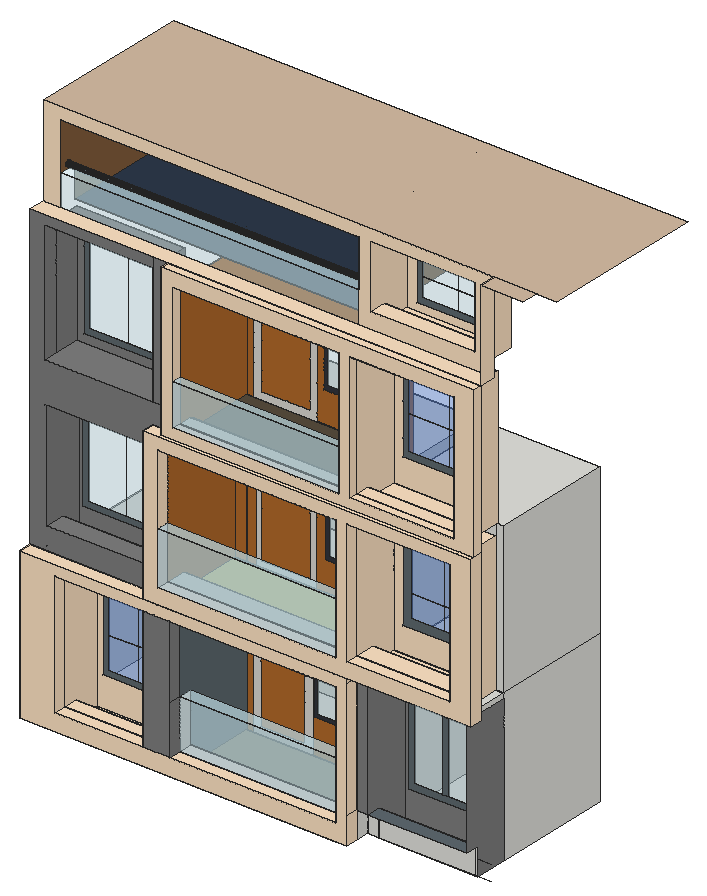
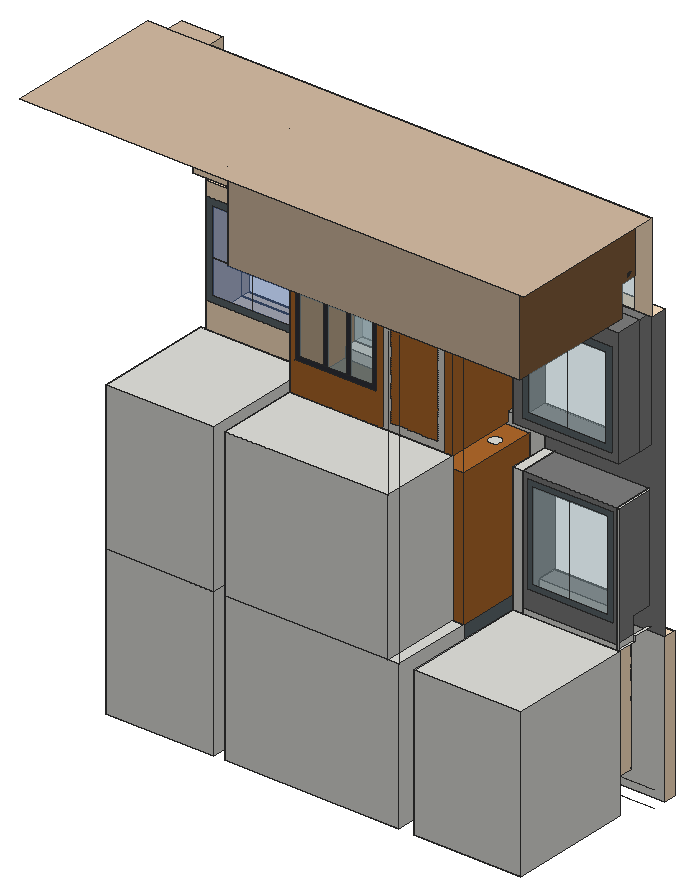
# SketchUp Ruby script. Lengths in inches.
U = 1.inch
M = Sketchup.active_model
def pt(a) = Geom::Point3d.new(a.map { |v| v * U })
def face(e, loops, mat)
  f = e.add_face(loops[0].map { |a| pt(a) })
  loops[1..].each { |l| e.add_face(l.map { |a| pt(a) }).erase! }
  f.material = f.back_material = mat if mat
  f
end
# faces: each face lists its corners as indices into pts; further lists are holes
def faces(e, pts, list, mat = nil) = list.each { |f| face(e, (f[0].is_a?(Array) ? f : [f]).map { |l| l.map { |i| pts[i] } }, mat) }
# xy, xz, yz: faces in a plane at the given z, y or x. An outline is a flat list of corners, or four numbers for a rectangle; further outlines are holes
def ring(l) = l.size == 4 ? [[l[0], l[1]], [l[2], l[1]], [l[2], l[3]], [l[0], l[3]]] : l.each_slice(2).to_a
def flat(e, list, mat, &to3) = list.each { |f| face(e, (f[0].is_a?(Array) ? f : [f]).map { |l| ring(l).map { |u, v| to3.(u, v) } }, mat) }
def xy(e, z, list, mat = nil) = flat(e, list, mat) { |x, y| [x, y, z] }
def xz(e, y, list, mat = nil) = flat(e, list, mat) { |x, z| [x, y, z] }
def yz(e, x, list, mat = nil) = flat(e, list, mat) { |y, z| [x, y, z] }
def lines(e, pts, list) = list.each { |a, b| e.add_line(pt(pts[a]), pt(pts[b])) }
# prism: a flat outline (further loops are holes) pulled along v
def prism(e, loops, v, mat = nil)
  f = face(e, loops, mat); d = Geom::Vector3d.new(v.map { |x| x * U })
  f.pushpull(f.normal.samedirection?(d) ? d.length : -d.length)
end
def box(e, o, s, mat = nil) = prism(e, [[o, [o[0] + s[0], o[1], o[2]], [o[0] + s[0], o[1] + s[1], o[2]], [o[0], o[1] + s[1], o[2]]]], [0, 0, s[2]], mat)
def at(x, y, z, deg = 0) = Geom::Transformation.translation(pt([x, y, z])) * Geom::Transformation.rotation(ORIGIN, Z_AXIS, deg.degrees)
def axes(o, x, y, z) = Geom::Transformation.new([*x, 0, *y, 0, *z, 0, *pt(o).to_a, 1])
def part(name) = M.definitions.add(name)
# library, detail: a bought-in or finely detailed component or shape, given as its bounding box
def library(name, o, s) = part(name).tap { |d| box(d.entities, o, s) }
def detail(e, o, s) = box(e.add_group.entities, o, s)
def put(e, d, t, mat = nil) = e.add_instance(d, t).tap { |i| i.material = mat if mat }
def group(e, t, mat = nil) = e.add_group.tap { |g| g.transformation = t; g.material = mat if mat }.entities
root = M.entities
M.materials.add("[0012_Bisque]").color = [255, 228, 196]
M.materials.add("[Blinds Wood Bamboo]").color = [131, 94, 60]
M.materials.add("[Carpet Diamond Olive]").color = [87, 77, 61]
M.materials.add("[Carpet Diamond Yellow]").color = [226, 217, 124]
M.materials.add("[Carpet Pattern Squares Multi]").color = [138, 129, 101]
M.materials.add("[Formica Laminate Dark]").color = [50, 53, 60]
M.materials.add("[Formica Laminate Light]").color = [213, 189, 164]
M.materials.add("[Formica Speckled Grey]").color = [94, 105, 111]
M.materials.add("[Leather Blue]").color = [45, 57, 74]
M.materials.add("[Slate Light Tile]").color = [127, 127, 127]
M.materials.add("[Terrazzo Tile Light]").color = [219, 217, 210]
M.materials.add("[Translucent Glass Blue]").color = [100, 149, 237]
M.materials["[Translucent Glass Blue]"].alpha = 0.5
M.materials.add("[Translucent Glass Safety]").color = [204, 235, 244]
M.materials["[Translucent Glass Safety]"].alpha = 0.5
M.materials.add("[Wood Bamboo]").color = [177, 105, 43]
xy(root,261,[[88.29,172.05,340.5,181.99],[340.5,172.05,349.51,181.99],[349.51,192.98,358.38,218.5],[99.28,214.18,186.23,314.81],[349.51,218.5,437.4,314.81],
  [198.44,249.06,340.5,314.81]])
xy(root,261,[[116.04,192.98,186.23,214.18]],"[0012_Bisque]")
xy(root,261,[[207.7,192.98,340.5,249.06]],"[Carpet Pattern Squares Multi]")
xy(root,261,[[358.38,192.98,437.4,218.5]],"[Formica Speckled Grey]")
xy(root,274.625,[[186.23,172.05,207.7,192.98],[207.7,181.99,340.5,192.98]])
xy(root,274.625,[[116.04,172.05,186.23,181.99],[207.7,172.05,340.5,181.99],[116.04,181.99,186.23,192.98]],"[0012_Bisque]")
xy(root,282.375,[[349.51,181.99,358.38,192.98]])
xy(root,282.375,[[358.38,181.99,437.4,192.98]],"[Formica Speckled Grey]")
xy(root,313.9375,[[207.7,181.99,340.5,192.98]],"[Translucent Glass Safety]")
xy(root,372.1875,[[222.36,205.33,221.21,205.48,220.14,205.93,219.22,206.63,218.51,207.55,218.07,208.62,217.92,209.77,218.07,210.92,218.51,211.99,219.22,212.91,220.14,213.61,221.21,214.05,222.36,214.21,223.51,214.05,224.58,213.61,225.5,212.91,226.2,211.99,226.64,210.92,226.8,209.77,226.64,208.62,226.2,207.55,225.5,206.63,224.58,205.93,223.51,205.48],[268.8,205.33,267.65,205.48,266.58,205.93,265.66,206.63,264.95,207.55,264.51,208.62,264.36,209.77,264.51,210.92,264.95,211.99,265.66,212.91,266.58,213.61,267.65,214.05,268.8,214.21,269.94,214.05,271.01,213.61,271.93,212.91,272.64,211.99,273.08,210.92,273.23,209.77,273.08,208.62,272.64,207.55,271.93,206.63,271.01,205.93,269.94,205.48],[320.23,205.33,319.08,205.48,318.01,205.93,317.1,206.63,316.39,207.55,315.95,208.62,315.8,209.77,315.95,210.92,316.39,211.99,317.1,212.91,318.01,213.61,319.08,214.05,320.23,214.21,321.38,214.05,322.45,213.61,323.37,212.91,324.08,211.99,324.52,210.92,324.67,209.77,324.52,208.62,324.08,207.55,323.37,206.63,322.45,205.93,321.38,205.48]])
xy(root,372.1875,[[116.04,172.05,186.23,181.99],[207.7,172.05,340.5,181.99],[116.04,181.99,186.23,214.18]],"[0012_Bisque]")
xy(root,372.1875,[[[207.7,181.99,340.5,249.06],[320.23,205.33,321.38,205.48,322.45,205.93,323.37,206.63,324.08,207.55,324.52,208.62,324.67,209.77,324.52,210.92,324.08,211.99,323.37,212.91,322.45,213.61,321.38,214.05,320.23,214.21,319.08,214.05,318.01,213.61,317.1,212.91,316.39,211.99,315.95,210.92,315.8,209.77,315.95,208.62,316.39,207.55,317.1,206.63,318.01,205.93,319.08,205.48],[222.36,205.33,223.51,205.48,224.58,205.93,225.5,206.63,226.2,207.55,226.64,208.62,226.8,209.77,226.64,210.92,226.2,211.99,225.5,212.91,224.58,213.61,223.51,214.05,222.36,214.21,221.21,214.05,220.14,213.61,219.22,212.91,218.51,211.99,218.07,210.92,217.92,209.77,218.07,208.62,218.51,207.55,219.22,206.63,220.14,205.93,221.21,205.48],[268.8,205.33,269.94,205.48,271.01,205.93,271.93,206.63,272.64,207.55,273.08,208.62,273.23,209.77,273.08,210.92,272.64,211.99,271.93,212.91,271.01,213.61,269.94,214.05,268.8,214.21,267.65,214.05,266.58,213.61,265.66,212.91,264.95,211.99,264.51,210.92,264.36,209.77,264.51,208.62,264.95,207.55,265.66,206.63,266.58,205.93,267.65,205.48]]],"[Wood Bamboo]")
xy(root,376.82,[[349.51,181.99,358.38,218.5]])
xy(root,376.82,[[358.38,181.99,437.4,218.5]],"[Slate Light Tile]")
xy(root,381,[[186.23,171.93,198.44,172.05],[198.44,171.93,340.5,172.05],[186.23,172.05,198.44,181.99],[198.44,172.05,340.5,181.99],[340.5,172.05,349.51,181.99],
  [198.44,181.99,431.53,198.09],[431.53,181.99,437.4,198.09],[99.8,198.09,101.61,214.18],[178.3,198.09,186.23,214.18],[431.53,198.09,437.4,218.5],
  [99.28,214.18,186.23,314.81],[349.51,218.5,437.4,314.81],[198.44,249.06,207.7,314.81],[207.7,249.06,340.5,314.81]])
xy(root,381,[[340.5,171.93,340.5,172.05,349.51,172.05,349.51,181.99,431.53,181.99,431.53,171.93],[431.53,171.93,437.4,181.99],[437.4,171.93,448.4,181.99],[88.29,172.05,186.23,181.99],[349.51,198.09,431.53,218.5]],"[0012_Bisque]")
xy(root,381,[[198.44,198.09,340.5,249.06]],"[Carpet Diamond Yellow]")
xy(root,384.875,[[99.8,181.99,101.61,198.09],[178.3,181.99,186.23,198.09]])
xy(root,384.875,[[101.61,198.09,178.3,214.18]],"[Slate Light Tile]")
xy(root,392.9375,[[198.44,171.93,340.5,181.99],[198.44,181.99,340.5,198.09]])
xy(root,392.9375,[[349.51,171.93,431.53,181.99],[349.51,181.99,431.53,198.09]],"[0012_Bisque]")
xy(root,399.125,[[101.61,181.99,178.3,198.09]],"[Slate Light Tile]")
xy(root,435,[[198.44,171.93,340.5,181.99]],"[Translucent Glass Safety]")
xy(root,485.17,[[99.8,181.99,101.61,214.18],[178.3,181.99,186.23,214.18]])
xy(root,485.17,[[101.61,181.99,178.3,214.18]],"[Slate Light Tile]")
xy(root,491.69,[[209.48,199,208.35,199.15,207.29,199.58,206.38,200.28,205.6875,201.1875,205.25,202.24,205.1,203.375,205.25,204.51,205.6875,205.5625,206.38,206.47,207.29,207.16,208.35,207.6,209.48,207.75,210.61,207.6,211.67,207.16,212.57,206.47,213.27,205.5625,213.7,204.51,213.85,203.375,213.7,202.24,213.27,201.1875,212.57,200.28,211.67,199.58,210.61,199.15],[260.29,199,259.16,199.15,258.1,199.58,257.2,200.28,256.5,201.1875,256.06,202.24,255.92,203.375,256.06,204.51,256.5,205.5625,257.2,206.47,258.1,207.16,259.16,207.6,260.29,207.75,261.42,207.6,262.48,207.16,263.38,206.47,264.08,205.5625,264.52,204.51,264.67,203.375,264.52,202.24,264.08,201.1875,263.38,200.28,262.48,199.58,261.42,199.15],[317.04,199,315.91,199.15,314.85,199.58,313.95,200.28,313.25,201.1875,312.81,202.24,312.67,203.375,312.81,204.51,313.25,205.5625,313.95,206.47,314.85,207.16,315.91,207.6,317.04,207.75,318.17,207.6,319.23,207.16,320.13,206.47,320.83,205.5625,321.27,204.51,321.42,203.375,321.27,202.24,320.83,201.1875,320.13,200.28,319.23,199.58,318.17,199.15]])
xy(root,491.69,[[198.44,171.93,340.5,181.99],[349.51,171.93,431.53,181.99],[349.51,181.99,431.53,218.5]],"[0012_Bisque]")
xy(root,491.69,[[[198.44,181.99,340.5,249.06],[209.48,199,210.61,199.15,211.67,199.58,212.57,200.28,213.27,201.1875,213.7,202.24,213.85,203.375,213.7,204.51,213.27,205.5625,212.57,206.47,211.67,207.16,210.61,207.6,209.48,207.75,208.35,207.6,207.29,207.16,206.38,206.47,205.6875,205.5625,205.25,204.51,205.1,203.375,205.25,202.24,205.6875,201.1875,206.38,200.28,207.29,199.58,208.35,199.15],[317.04,199,318.17,199.15,319.23,199.58,320.13,200.28,320.83,201.1875,321.27,202.24,321.42,203.375,321.27,204.51,320.83,205.5625,320.13,206.47,319.23,207.16,318.17,207.6,317.04,207.75,315.91,207.6,314.85,207.16,313.95,206.47,313.25,205.5625,312.81,204.51,312.67,203.375,312.81,202.24,313.25,201.1875,313.95,200.28,314.85,199.58,315.91,199.15],[260.29,199,261.42,199.15,262.48,199.58,263.38,200.28,264.08,201.1875,264.52,202.24,264.67,203.375,264.52,204.51,264.08,205.5625,263.38,206.47,262.48,207.16,261.42,207.6,260.29,207.75,259.16,207.6,258.1,207.16,257.2,206.47,256.5,205.5625,256.06,204.51,255.92,203.375,256.06,202.24,256.5,201.1875,257.2,200.28,258.1,199.58,259.16,199.15]]],"[Wood Bamboo]")
xy(root,501,[[198.44,175.18,437.4,181.99],[437.4,175.18,448.4,181.99],[349.51,218.5,437.4,314.81],[207.7,249.06,340.5,314.81]])
xy(root,501,[[186.23,171.93,198.44,181.99],[198.44,171.93,437.4,175.18],[437.4,171.93,448.4,175.18],[349.51,193.01,431.53,218.5],[431.53,193.01,432.73,218.5]],"[0012_Bisque]")
xy(root,501,[[207.7,193.01,340.5,249.06]],"[Carpet Diamond Olive]")
xy(root,509,[[207.7,175.18,340.5,181.99],[207.7,181.99,340.5,193.01]])
xy(root,509,[[349.51,175.18,432.73,181.99],[349.51,181.99,432.73,193.01]],"[0012_Bisque]")
xy(root,517.375,[[99.8,181.99,186.23,214.18]],"[Slate Light Tile]")
xy(root,542.5,[[207.7,175.18,340.5,181.99]],"[Translucent Glass Safety]")
xy(root,609.93,[[226.8,191.29,225.88,191.42,225.02,191.77,224.28,192.34,223.72,193.08,223.36,193.93,223.24,194.86,223.36,195.78,223.72,196.64,224.28,197.375,225.02,197.94,225.88,198.3,226.8,198.42,227.73,198.3,228.58,197.94,229.32,197.375,229.89,196.64,230.24,195.78,230.37,194.86,230.24,193.93,229.89,193.08,229.32,192.34,228.58,191.77,227.73,191.42],[275.55,191.29,274.63,191.42,273.77,191.77,273.03,192.34,272.47,193.08,272.11,193.93,271.99,194.86,272.11,195.78,272.47,196.64,273.03,197.375,273.77,197.94,274.63,198.3,275.55,198.42,276.48,198.3,277.33,197.94,278.07,197.375,278.64,196.64,278.99,195.78,279.12,194.86,278.99,193.93,278.64,193.08,278.07,192.34,277.33,191.77,276.48,191.42],[316.55,191.29,315.63,191.42,314.77,191.77,314.03,192.34,313.47,193.08,313.11,193.93,312.99,194.86,313.11,195.78,313.47,196.64,314.03,197.375,314.77,197.94,315.63,198.3,316.55,198.42,317.48,198.3,318.33,197.94,319.07,197.375,319.64,196.64,319.99,195.78,320.12,194.86,319.99,193.93,319.64,193.08,319.07,192.34,318.33,191.77,317.48,191.42]])
xy(root,609.93,[[207.7,175.18,340.5,181.99]],"[0012_Bisque]")
xy(root,609.93,[[[207.7,181.99,340.5,249.06],[316.55,191.29,317.48,191.42,318.33,191.77,319.07,192.34,319.64,193.08,319.99,193.93,320.12,194.86,319.99,195.78,319.64,196.64,319.07,197.375,318.33,197.94,317.48,198.3,316.55,198.42,315.63,198.3,314.77,197.94,314.03,197.375,313.47,196.64,313.11,195.78,312.99,194.86,313.11,193.93,313.47,193.08,314.03,192.34,314.77,191.77,315.63,191.42],[226.8,191.29,227.73,191.42,228.58,191.77,229.32,192.34,229.89,193.08,230.24,193.93,230.37,194.86,230.24,195.78,229.89,196.64,229.32,197.375,228.58,197.94,227.73,198.3,226.8,198.42,225.88,198.3,225.02,197.94,224.28,197.375,223.72,196.64,223.36,195.78,223.24,194.86,223.36,193.93,223.72,193.08,224.28,192.34,225.02,191.77,225.88,191.42],[275.55,191.29,276.48,191.42,277.33,191.77,278.07,192.34,278.64,193.08,278.99,193.93,279.12,194.86,278.99,195.78,278.64,196.64,278.07,197.375,277.33,197.94,276.48,198.3,275.55,198.42,274.63,198.3,273.77,197.94,273.03,197.375,272.47,196.64,272.11,195.78,271.99,194.86,272.11,193.93,272.47,193.08,273.03,192.34,273.77,191.77,274.63,191.42]]],"[Wood Bamboo]")
xy(root,610.28,[[349.51,175.18,432.73,181.99],[349.51,181.99,432.73,218.5]],"[0012_Bisque]")
xy(root,613.53,[[99.8,181.99,186.23,193.01],[99.8,193.01,186.23,214.18]],"[Slate Light Tile]")
xy(root,621,[[198.44,175.18,448.4,181.99],[88.29,181.99,448.4,195.54],[349.51,209.22,432.73,231.625]],"[0012_Bisque]")
xy(root,621,[[101.84,209.22,340.5,312.25]],"[Leather Blue]")
xy(root,633.5,[[349.51,195.54,432.73,209.22]],"[0012_Bisque]")
xy(root,645.8125,[[101.84,195.54,340.5,209.22]],"[Translucent Glass Safety]")
xy(root,683.72,[[126.93,241.64,125.08,241.88,123.37,242.59,121.89,243.72,120.76,245.2,120.05,246.92,119.8,248.76,120.05,250.61,120.76,252.33,121.89,253.8,123.37,254.93,125.08,255.64,126.93,255.89,128.77,255.64,130.49,254.93,131.97,253.8,133.1,252.33,133.8125,250.61,134.05,248.76,133.8125,246.92,133.1,245.2,131.97,243.72,130.49,242.59,128.77,241.88],[220.12,241.64,218.27,241.88,216.55,242.59,215.08,243.72,213.95,245.2,213.23,246.92,212.99,248.76,213.23,250.61,213.95,252.33,215.08,253.8,216.55,254.93,218.27,255.64,220.12,255.89,221.96,255.64,223.68,254.93,225.15,253.8,226.29,252.33,227,250.61,227.24,248.76,227,246.92,226.29,245.2,225.15,243.72,223.68,242.59,221.96,241.88],[310.74,241.64,308.9,241.88,307.18,242.59,305.7,243.72,304.57,245.2,303.86,246.92,303.62,248.76,303.86,250.61,304.57,252.33,305.7,253.8,307.18,254.93,308.9,255.64,310.74,255.89,312.59,255.64,314.3,254.93,315.78,253.8,316.91,252.33,317.625,250.61,317.87,248.76,317.625,246.92,316.91,245.2,315.78,243.72,314.3,242.59,312.59,241.88]])
xy(root,683.72,[[349.51,195.54,432.73,231.625]],"[0012_Bisque]")
xy(root,683.72,[[[101.84,195.54,340.5,312.25],[126.93,241.64,128.77,241.88,130.49,242.59,131.97,243.72,133.1,245.2,133.8125,246.92,134.05,248.76,133.8125,250.61,133.1,252.33,131.97,253.8,130.49,254.93,128.77,255.64,126.93,255.89,125.08,255.64,123.37,254.93,121.89,253.8,120.76,252.33,120.05,250.61,119.8,248.76,120.05,246.92,120.76,245.2,121.89,243.72,123.37,242.59,125.08,241.88],[310.74,241.64,312.59,241.88,314.3,242.59,315.78,243.72,316.91,245.2,317.625,246.92,317.87,248.76,317.625,250.61,316.91,252.33,315.78,253.8,314.3,254.93,312.59,255.64,310.74,255.89,308.9,255.64,307.18,254.93,305.7,253.8,304.57,252.33,303.86,250.61,303.62,248.76,303.86,246.92,304.57,245.2,305.7,243.72,307.18,242.59,308.9,241.88],[220.12,241.64,221.96,241.88,223.68,242.59,225.15,243.72,226.29,245.2,227,246.92,227.24,248.76,227,250.61,226.29,252.33,225.15,253.8,223.68,254.93,221.96,255.64,220.12,255.89,218.27,255.64,216.55,254.93,215.08,253.8,213.95,252.33,213.23,250.61,212.99,248.76,213.23,246.92,213.95,245.2,215.08,243.72,216.55,242.59,218.27,241.88]]],"[Blinds Wood Bamboo]")
xy(root,693,[[448.4,181.99,482.08,195.54],[88.29,195.54,498.52,325.8]],"[Formica Laminate Light]")
xz(root,171.93,[[[186.23,381,448.4,501],[198.44,392.9375,340.5,491.69],[349.51,392.9375,431.53,491.69]]],"[0012_Bisque]")
xz(root,171.93,[[198.44,392.9375,340.5,435]],"[Translucent Glass Safety]")
xz(root,172.05,[[[88.29,261,349.51,381],[116.04,274.625,340.5,372.1875]]],"[0012_Bisque]")
xz(root,172.05,[[186.23,274.625,207.7,372.1875]],"[Slate Light Tile]")
xz(root,175.18,[[[198.44,501,448.4,621],[207.7,509,340.5,609.93],[349.51,509,432.73,610.28]]],"[0012_Bisque]")
xz(root,175.18,[[207.7,509,340.5,542.5]],"[Translucent Glass Safety]")
xz(root,181.99,[[[88.29,261,349.51,381],[207.7,274.625,340.5,372.1875],[116.04,274.625,186.23,372.1875]],[[186.23,381,448.4,501],[198.44,392.9375,340.5,491.69],[349.51,392.9375,431.53,491.69]],[[198.44,501,448.4,621],[207.7,509,340.5,609.93],[349.51,509,432.73,610.28]]])
xz(root,181.99,[[349.51,282.375,358.38,376.82],[349.51,376.82,437.4,381],[88.29,381,186.23,381,186.23,384.875,178.3,384.875,178.3,399.125,101.61,399.125,101.61,485.17,186.23,485.17,186.23,501,198.44,501,198.44,517.375,99.8,517.375,99.8,613.53,186.23,613.53,186.23,621,88.29,621],[178.3,384.875,186.23,485.17],[186.23,517.375,198.44,621]],"[Slate Light Tile]")
xz(root,181.99,[[207.7,274.625,340.5,313.9375],[198.44,392.9375,340.5,435],[207.7,509,340.5,542.5]],"[Translucent Glass Safety]")
xz(root,192.98,[[116.04,261,186.23,274.625],[186.23,261,207.7,274.625],[207.7,261,340.5,274.625],[349.51,261,358.38,282.375],[358.38,261,434.83,282.375],
  [434.83,261,437.4,282.375]])
xz(root,192.98,[[207.7,274.625,340.5,313.9375]],"[Translucent Glass Safety]")
xz(root,193.01,[[207.7,501,340.5,509],[431.53,501,432.73,509]])
xz(root,193.01,[[349.51,501,431.53,509]],"[0012_Bisque]")
xz(root,195.54,[[[88.29,621,101.84,621,101.84,683.72,340.5,683.72,340.5,621,448.4,621,448.4,693,88.29,693],[349.51,633.5,432.73,683.72]]],"[0012_Bisque]")
xz(root,195.54,[[101.84,621,340.5,645.8125]],"[Translucent Glass Safety]")
xz(root,198.09,[[99.8,381,101.61,384.875],[178.3,381,186.23,384.875],[198.44,381,340.5,392.9375],[340.5,381,349.51,392.9375],[101.61,384.875,178.3,399.125]])
xz(root,198.09,[[349.51,381,431.53,392.9375]],"[0012_Bisque]")
xz(root,209.22,[[349.51,621,432.73,633.5]],"[0012_Bisque]")
xz(root,209.22,[[101.84,621,340.5,645.8125]],"[Translucent Glass Safety]")
xz(root,214.18,[[99.28,261,99.28,381,186.23,381,186.23,372.1875,116.04,372.1875,116.04,358.83,114.09,358.83,114.09,284.52,116.04,284.52,116.04,261],[114.09,284.52,116.04,358.83],[99.8,381,101.61,485.17],[101.61,381,178.3,384.875],[178.3,381,186.23,485.17]])
xz(root,214.18,[[[116.04,261,186.23,372.1875],[120.92,284.51,178.24,359.76]]],"[0012_Bisque]")
xz(root,214.18,[[[120.92,284.51,178.24,359.76],[125.41,289,173.75,355.28]],[[104.95,400.15,174.13,480.77],[109.22,404.43,169.85,476.49]],[[105.43,523.82,178.05,600.88],[110.47,528.86,173.01,595.84]]],"[Formica Speckled Grey]")
xz(root,214.18,[[[101.61,384.875,178.3,485.17],[104.95,400.15,174.13,480.77]],[[99.8,517.375,186.23,613.53],[105.43,523.82,178.05,600.88]]],"[Slate Light Tile]")
xz(root,214.18,[[125.41,289,149.58,314.58],[149.58,289,173.75,314.58],[125.41,314.58,149.58,355.28],[149.58,314.58,173.75,355.28]],"[Translucent Glass Blue]")
xz(root,214.18,[[109.22,404.43,139.54,476.49],[139.54,404.43,169.85,476.49],[110.47,528.86,141.74,595.84],[141.74,528.86,173.01,595.84]],"[Translucent Glass Safety]")
xz(root,218.5,[[349.51,261,358.38,376.82],[349.51,376.82,437.4,381],[431.53,381,437.4,501],[349.51,491.69,431.53,501]])
xz(root,218.5,[[[349.51,381,431.53,491.69],[357.125,401.3125,423.9375,476.5]],[349.51,501,432.73,501,432.73,522.05,356.73,522.05,356.73,598.05,432.73,598.05,432.73,610.28,349.51,610.28]],"[0012_Bisque]")
xz(root,218.5,[[[361.62,286.07,422.24,362.07],[366.86,291.3125,416.99,356.82]],[389.17,291.3125,393.55,356.82],[[357.125,401.3125,423.9375,476.5],[364,408.19,417.0625,469.625]],[[356.73,522.05,432.73,598.05],[361.96,527.28,427.49,592.81]]],"[Formica Speckled Grey]")
xz(root,218.5,[[[358.38,261,437.4,376.82],[361.62,286.07,422.24,362.07]]],"[Slate Light Tile]")
xz(root,218.5,[[364,408.19,390.53,426],[390.53,408.19,417.0625,426],[364,426,390.53,469.625],[390.53,426,417.0625,469.625],[361.96,527.28,394.73,554.52],
  [394.73,527.28,427.49,554.52],[361.96,554.52,394.73,592.81],[394.73,554.52,427.49,592.81]],"[Translucent Glass Blue]")
xz(root,218.5,[[366.86,291.3125,389.17,356.82],[393.55,291.3125,416.99,356.82]],"[Translucent Glass Safety]")
xz(root,231.625,[[[349.51,621,432.73,683.72],[357.63,626.77,423.94,679.02]]],"[0012_Bisque]")
xz(root,231.625,[[[357.63,626.77,423.94,679.02],[362.47,631.61,419.1,674.17]]],"[Formica Speckled Grey]")
xz(root,231.625,[[362.47,631.61,390.79,646.95],[390.79,631.61,419.1,646.95],[362.47,646.95,390.79,674.17],[390.79,646.95,419.1,674.17]],"[Translucent Glass Safety]")
xz(root,249.06,[[198.44,261,207.7,261,207.7,372.1875,340.5,372.1875,340.5,381,198.44,381],[207.7,491.69,340.5,501]])
xz(root,249.06,[[[262.39,289.15,335.64,357.34],[264.89,291.66,333.13,354.84]],[279.62,291.66,281.95,354.84],[299.01,291.66,301.34,354.84],[316.57,291.66,318.91,354.84],[[270.07,403.99,336.38,473.49],[274,407.92,332.45,469.55]],
  [291.97,407.92,295.12,469.55],[311.91,407.92,315.05,469.55],[[268.94,525.92,335.82,598.36],[272.67,529.65,332.09,594.63]],[290.18,529.65,293.6,594.63],[309.42,529.65,312.85,594.63]],"[Formica Laminate Dark]")
xz(root,249.06,[[[212.99,261,260.24,354.1875],[218.83,266.84,254.4,348.35]],[[214.77,381,263.71,474.6875],[220.03,386.25,258.46,469.43]],[[213.59,501,264.03,599.625],[219.74,507.14,257.89,593.48]]],"[Terrazzo Tile Light]")
xz(root,249.06,[[264.89,291.66,279.62,354.84],[281.95,291.66,299.01,354.84],[301.34,291.66,316.57,354.84],[318.91,291.66,333.13,354.84],[274,407.92,291.97,469.55],
  [295.12,407.92,311.91,469.55],[315.05,407.92,332.45,469.55],[272.67,529.65,290.18,594.63],[293.6,529.65,309.42,594.63],[312.85,529.65,332.09,594.63]],"[Translucent Glass Safety]")
xz(root,249.06,[[[207.7,261,212.99,261,212.99,354.1875,260.24,354.1875,260.24,261,340.5,261,340.5,372.1875,207.7,372.1875],[262.39,289.15,335.64,357.34]],[218.83,266.84,254.4,348.35],[198.44,381,207.7,491.69],[[207.7,381,214.77,381,214.77,474.6875,263.71,474.6875,263.71,381,340.5,381,340.5,491.69,207.7,491.69],[270.07,403.99,336.38,473.49]],[220.03,386.25,258.46,469.43],
  [[207.7,501,213.59,501,213.59,599.625,264.03,599.625,264.03,501,340.5,501,340.5,609.93,207.7,609.93],[268.94,525.92,335.82,598.36]],[219.74,507.14,257.89,593.48]],"[Wood Bamboo]")
xz(root,312.25,[[101.84,621,340.5,683.72]],"[Formica Laminate Light]")
xz(root,314.81,[[99.28,261,186.23,381],[198.44,261,340.5,381],[349.51,261,437.4,381],[207.7,381,340.5,501],[349.51,381,437.4,501]])
yz(root,88.29,[[172.05,261,181.99,381]],"[0012_Bisque]")
yz(root,99.28,[[214.18,261,314.81,381]])
yz(root,99.8,[[181.99,517.375,193.01,613.53],[193.01,517.375,214.18,613.53]],"[Slate Light Tile]")
yz(root,101.61,[[198.09,381,214.18,384.875]])
yz(root,101.61,[[198.09,384.875,214.18,384.875,214.18,485.17,181.99,485.17,181.99,399.125,198.09,399.125]],"[Slate Light Tile]")
yz(root,101.84,[[[209.22,621,312.25,621,312.25,683.72,195.54,683.72,195.54,645.8125,209.22,645.8125],[201.64,648.1,201.14,648.17,200.67,648.36,200.27,648.67,199.96,649.07,199.77,649.54,199.7,650.04,199.77,650.54,199.96,651.01,200.27,651.41,200.67,651.72,201.14,651.91,201.64,651.98,202.14,651.91,202.61,651.72,203.01,651.41,203.32,651.01,203.51,650.54,203.58,650.04,203.51,649.54,203.32,649.07,203.01,648.67,202.61,648.36,202.14,648.17]]],"[Blinds Wood Bamboo]")
yz(root,116.04,[[192.98,261,214.18,261,214.18,372.1875,181.99,372.1875,181.99,274.625,192.98,274.625],[172.05,274.625,181.99,372.1875]],"[0012_Bisque]")
yz(root,178.3,[[198.09,381,214.18,384.875],[181.99,384.875,198.09,399.125]])
yz(root,178.3,[[198.09,384.875,198.09,399.125,181.99,399.125,181.99,485.17,214.18,485.17,214.18,384.875]],"[Slate Light Tile]")
yz(root,186.23,[[214.18,261,314.81,381],[171.93,381,181.99,384.875],[198.09,381,214.18,381,214.18,485.17,181.99,485.17,181.99,384.875,198.09,384.875]])
yz(root,186.23,[[192.98,261,192.98,274.625,181.99,274.625,181.99,372.1875,214.18,372.1875,214.18,261],[171.93,384.875,181.99,485.17],[171.93,485.17,181.99,501]],"[0012_Bisque]")
yz(root,186.23,[[172.05,274.625,181.99,372.1875],[181.99,517.375,214.18,613.53]],"[Slate Light Tile]")
yz(root,198.44,[[249.06,261,314.81,381],[171.93,392.9375,181.99,435]])
yz(root,198.44,[[171.93,435,181.99,491.69],[175.18,501,181.99,517.375],[175.18,517.375,181.99,621]],"[0012_Bisque]")
yz(root,198.44,[[198.09,381,249.06,381,249.06,491.69,181.99,491.69,181.99,392.9375,198.09,392.9375]],"[Wood Bamboo]")
yz(root,207.7,[[181.99,274.625,192.98,313.9375],[249.06,381,314.81,501],[175.18,509,181.99,542.5]])
yz(root,207.7,[[175.18,542.5,181.99,609.93]],"[0012_Bisque]")
yz(root,207.7,[[192.98,261,249.06,261,249.06,372.1875,181.99,372.1875,181.99,313.9375,192.98,313.9375]],"[Formica Speckled Grey]")
yz(root,207.7,[[172.05,274.625,181.99,313.9375],[172.05,313.9375,181.99,372.1875]],"[Slate Light Tile]")
yz(root,207.7,[[193.01,501,249.06,501,249.06,609.93,181.99,609.93,181.99,509,193.01,509]],"[Wood Bamboo]")
yz(root,340.5,[[249.06,261,314.81,381],[172.05,274.625,181.99,313.9375],[181.99,274.625,192.98,313.9375],[249.06,381,314.81,501],[171.93,392.9375,181.99,435],
  [175.18,509,181.99,542.5],[201.64,648.1,202.14,648.17,202.61,648.36,203.01,648.67,203.32,649.07,203.51,649.54,203.58,650.04,203.51,650.54,203.32,651.01,203.01,651.41,202.61,651.72,202.14,651.91,201.64,651.98,201.14,651.91,200.67,651.72,200.27,651.41,199.96,651.01,199.77,650.54,199.7,650.04,199.77,649.54,199.96,649.07,200.27,648.67,200.67,648.36,201.14,648.17]])
yz(root,340.5,[[172.05,313.9375,181.99,372.1875],[171.93,435,181.99,491.69],[175.18,542.5,181.99,609.93],[[209.22,621,209.22,645.8125,195.54,645.8125,195.54,683.72,249.06,683.72,249.06,621],[201.64,648.1,202.14,648.17,202.61,648.36,203.01,648.67,203.32,649.07,203.51,649.54,203.58,650.04,203.51,650.54,203.32,651.01,203.01,651.41,202.61,651.72,202.14,651.91,201.64,651.98,201.14,651.91,200.67,651.72,200.27,651.41,199.96,651.01,199.77,650.54,199.7,650.04,199.77,649.54,199.96,649.07,200.27,648.67,200.67,648.36,201.14,648.17]]],"[0012_Bisque]")
yz(root,340.5,[[249.06,621,312.25,683.72]],"[Blinds Wood Bamboo]")
yz(root,340.5,[[192.98,261,192.98,313.9375,181.99,313.9375,181.99,372.1875,249.06,372.1875,249.06,261],[198.09,381,198.09,392.9375,181.99,392.9375,181.99,491.69,249.06,491.69,249.06,381],[193.01,501,193.01,509,181.99,509,181.99,609.93,249.06,609.93,249.06,501]],"[Wood Bamboo]")
yz(root,349.51,[[181.99,261,192.98,282.375],[192.98,261,192.98,282.375,181.99,282.375,181.99,376.82,218.5,376.82,218.5,261],[218.5,261,314.81,381],[218.5,381,314.81,501]])
yz(root,349.51,[[172.05,261,181.99,282.375],[172.05,282.375,181.99,376.82],[172.05,376.82,181.99,381],[198.09,381,218.5,381,218.5,491.69,181.99,491.69,181.99,392.9375,198.09,392.9375],[171.93,392.9375,181.99,491.69],
  [193.01,501,218.5,501,218.5,610.28,181.99,610.28,181.99,509,193.01,509],[175.18,509,181.99,610.28],[209.22,621,231.625,621,231.625,683.72,195.54,683.72,195.54,633.5,209.22,633.5]],"[0012_Bisque]")
yz(root,358.38,[[192.98,261,218.5,261,218.5,376.82,181.99,376.82,181.99,282.375,192.98,282.375]],"[Slate Light Tile]")
yz(root,431.53,[[198.09,381,198.09,392.9375,181.99,392.9375,181.99,491.69,218.5,491.69,218.5,381],[171.93,392.9375,181.99,491.69]],"[0012_Bisque]")
yz(root,432.73,[[193.01,501,193.01,509,181.99,509,181.99,610.28,218.5,610.28,218.5,501],[175.18,509,181.99,610.28],[209.22,621,209.22,633.5,195.54,633.5,195.54,683.72,231.625,683.72,231.625,621]],"[0012_Bisque]")
yz(root,437.4,[[218.5,261,314.81,381],[181.99,376.82,218.5,381],[218.5,381,314.81,501]])
yz(root,437.4,[[192.98,261,192.98,282.375,181.99,282.375,181.99,376.82,218.5,376.82,218.5,261]],"[Slate Light Tile]")
yz(root,448.4,[[171.93,381,181.99,501],[175.18,501,181.99,621],[181.99,621,195.54,693]],"[0012_Bisque]")
p = [[340.5,201.64,648.1],[340.5,201.14,648.17],[101.84,201.14,648.17],[101.84,201.64,648.1],[340.5,202.14,648.17],[101.84,202.14,648.17],
  [340.5,200.67,648.36],[101.84,200.67,648.36],[340.5,202.61,648.36],[101.84,202.61,648.36],[340.5,200.27,648.67],[101.84,200.27,648.67],
  [340.5,203.01,648.67],[101.84,203.01,648.67],[340.5,199.96,649.07],[101.84,199.96,649.07],[340.5,203.32,649.07],[101.84,203.32,649.07],
  [340.5,199.77,649.54],[101.84,199.77,649.54],[340.5,203.51,649.54],[101.84,203.51,649.54],[340.5,199.7,650.04],[101.84,199.7,650.04],
  [340.5,203.58,650.04],[101.84,203.58,650.04],[340.5,199.77,650.54],[101.84,199.77,650.54],[340.5,203.51,650.54],[101.84,203.51,650.54],
  [340.5,199.96,651.01],[101.84,199.96,651.01],[340.5,203.32,651.01],[101.84,203.32,651.01],[340.5,200.27,651.41],[101.84,200.27,651.41],
  [340.5,203.01,651.41],[101.84,203.01,651.41],[340.5,200.67,651.72],[101.84,200.67,651.72],[340.5,202.61,651.72],[101.84,202.61,651.72],
  [340.5,201.14,651.91],[101.84,201.14,651.91],[340.5,202.14,651.91],[101.84,202.14,651.91],[340.5,201.64,651.98],[101.84,201.64,651.98],
  [437.4,192.98,261],[448.4,192.98,261],[116.04,192.98,261],[88.29,192.98,261],[340.5,192.98,261],[340.5,181.99,261],
  [116.04,192.98,274.625],[88.29,192.98,274.625],[437.4,192.98,273.375],[448.4,192.98,273.375],[198.44,314.81,381],[198.44,314.81,621],
  [198.44,249.06,491.69],[198.44,249.06,621],[207.7,314.81,501],[207.7,314.81,621],[207.7,249.06,609.93],[207.7,249.06,621],
  [340.5,249.06,609.93],[340.5,249.06,621],[340.5,249.06,683.72],[340.5,249.06,693],[340.5,312.25,683.72],[340.5,312.25,693]]
faces(root,p,[[0,1,2,3],[4,0,3,5],[1,6,7,2],[8,4,5,9],[6,10,11,7],[12,8,9,13],[10,14,15,11],[16,12,13,17],
  [14,18,19,15],[20,16,17,21],[18,22,23,19],[24,20,21,25],[22,26,27,23],[28,24,25,29],[26,30,31,27],[32,28,29,33],
  [30,34,35,31],[36,32,33,37],[34,38,39,35],[40,36,37,41],[38,42,43,39],[44,40,41,45],[42,46,47,43],[46,44,45,47]],"[Formica Speckled Grey]")
lines(root,p,[[48,49],[50,51],[52,53],[54,55],[56,57],[58,59],[60,61],[62,63],[64,65],[66,67],[68,69],[70,71]])
